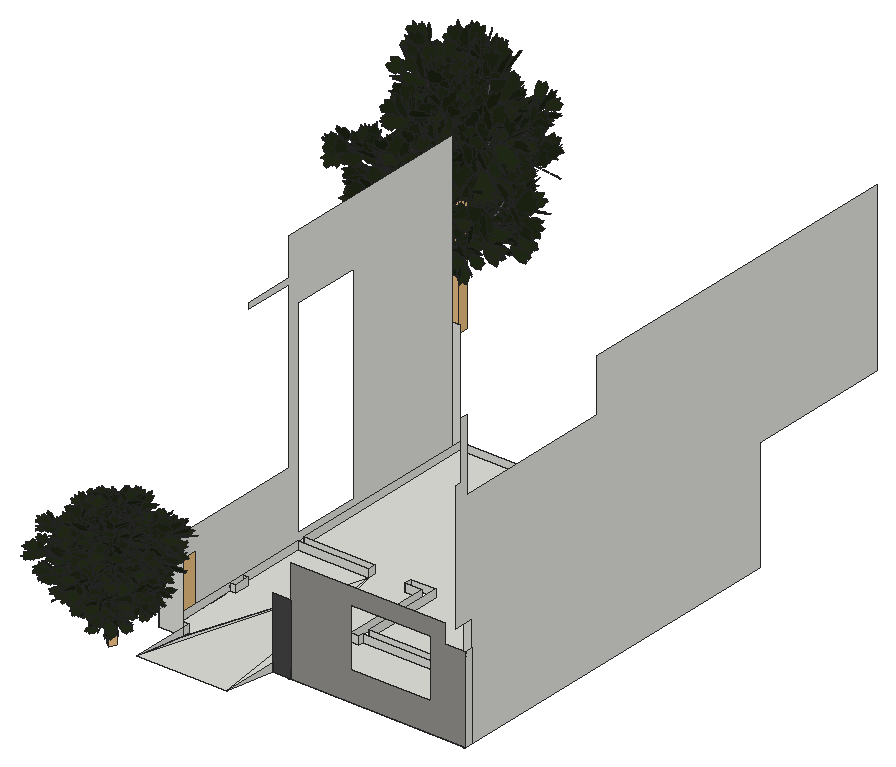
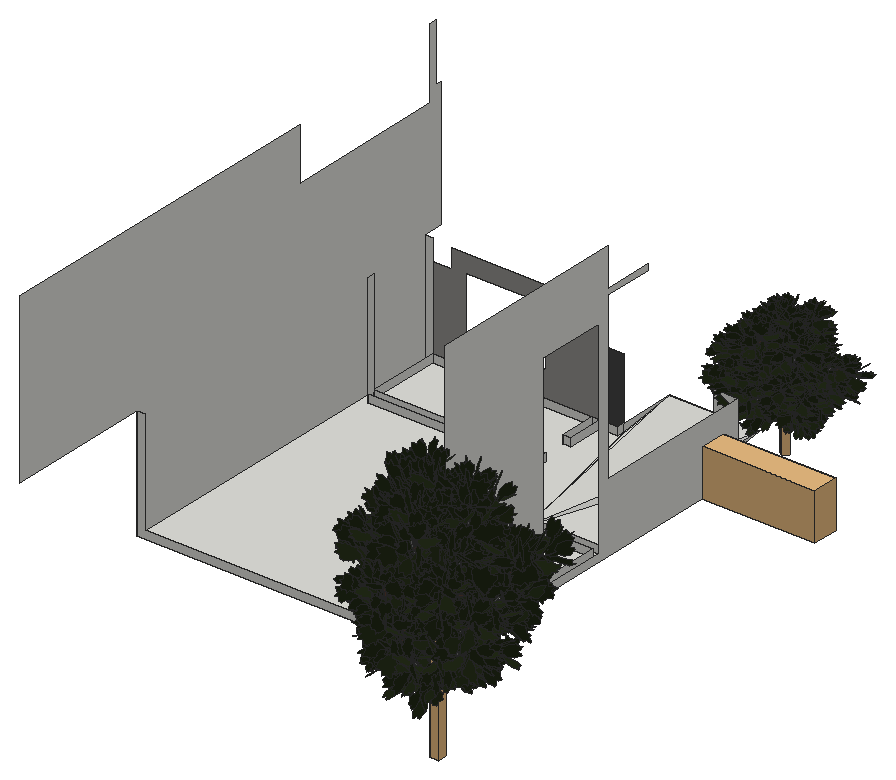
# SketchUp Ruby script. Lengths in inches.
U = 1.inch
M = Sketchup.active_model
def pt(a) = Geom::Point3d.new(a.map { |v| v * U })
def face(e, loops, mat)
  f = e.add_face(loops[0].map { |a| pt(a) })
  loops[1..].each { |l| e.add_face(l.map { |a| pt(a) }).erase! }
  f.material = f.back_material = mat if mat
  f
end
# faces: each face lists its corners as indices into pts; further lists are holes
def faces(e, pts, list, mat = nil) = list.each { |f| face(e, (f[0].is_a?(Array) ? f : [f]).map { |l| l.map { |i| pts[i] } }, mat) }
# xy, xz, yz: faces in a plane at the given z, y or x. An outline is a flat list of corners, or four numbers for a rectangle; further outlines are holes
def ring(l) = l.size == 4 ? [[l[0], l[1]], [l[2], l[1]], [l[2], l[3]], [l[0], l[3]]] : l.each_slice(2).to_a
def flat(e, list, mat, &to3) = list.each { |f| face(e, (f[0].is_a?(Array) ? f : [f]).map { |l| ring(l).map { |u, v| to3.(u, v) } }, mat) }
def xy(e, z, list, mat = nil) = flat(e, list, mat) { |x, y| [x, y, z] }
def xz(e, y, list, mat = nil) = flat(e, list, mat) { |x, z| [x, y, z] }
def yz(e, x, list, mat = nil) = flat(e, list, mat) { |y, z| [x, y, z] }
def lines(e, pts, list) = list.each { |a, b| e.add_line(pt(pts[a]), pt(pts[b])) }
# prism: a flat outline (further loops are holes) pulled along v
def prism(e, loops, v, mat = nil)
  f = face(e, loops, mat); d = Geom::Vector3d.new(v.map { |x| x * U })
  f.pushpull(f.normal.samedirection?(d) ? d.length : -d.length)
end
def box(e, o, s, mat = nil) = prism(e, [[o, [o[0] + s[0], o[1], o[2]], [o[0] + s[0], o[1] + s[1], o[2]], [o[0], o[1] + s[1], o[2]]]], [0, 0, s[2]], mat)
def at(x, y, z, deg = 0) = Geom::Transformation.translation(pt([x, y, z])) * Geom::Transformation.rotation(ORIGIN, Z_AXIS, deg.degrees)
def axes(o, x, y, z) = Geom::Transformation.new([*x, 0, *y, 0, *z, 0, *pt(o).to_a, 1])
def part(name) = M.definitions.add(name)
# library, detail: a bought-in or finely detailed component or shape, given as its bounding box
def library(name, o, s) = part(name).tap { |d| box(d.entities, o, s) }
def detail(e, o, s) = box(e.add_group.entities, o, s)
def put(e, d, t, mat = nil) = e.add_instance(d, t).tap { |i| i.material = mat if mat }
def group(e, t, mat = nil) = e.add_group.tap { |g| g.transformation = t; g.material = mat if mat }.entities
root = M.entities
M.materials.add("Green ash – green texture").color = [33, 41, 22]
M.materials.add("[Color_005]1").color = [114, 114, 114]
M.materials.add("[Color_D09]1").color = [86, 59, 49]
M.materials.add("[Granite Dark Gray]").color = [69, 68, 68]
M.materials.add("[Granite Light Gray]").color = [149, 148, 144]
c1 = library("Tree trunk",[-6.35,9.4375,-76.57],[12.56,13.68,315.77])
c2 = part("Component\#32")
xz(c2.entities,0,[[2.54,0,9.87,0.64,10.99,2.07,11.4,3.42,15.13,2.28,14.48,4.31,16.14,5.21,16.14,6.08,19.81,7.28,19.6,9.67,17.45,11.49,17.45,12.16,18.82,14.37,17.48,14.37,14.41,13.66,14.41,15.23,12.5625,17.49,9.84,15.21,8.9,13.85,7.74,13.625,7.35,12.68,6.87,13.02,6.35,12.27,5.92,10.47,4.2,7.42,2.84,6.89,0,2.38,0.07,1.59,2.8125,4.94,3.37,3.59,2.54,3.37,2.12,2.22]],"Green ash – green texture")
c3 = part("Component\#31")
xz(c3.entities,0,[[1.1,0,1.61,0,2.73,1.11,4.34,2.72,5.21,6.36,5.85,7.16,6.35,6.9375,6.85,8.05,8.03,8.05,8.625,9.25,10.11,11.7,9.56,13.83,9.56,15.84,7.83,15.84,6.03,14.37,5.31,16.54,4.4375,17.39,1.45,14.31,0,9.15,1.4,5.18,3.01,6.08,1.98,1.39]],"Green ash – green texture")
c4 = part("Component\#30")
put(c4.entities,c2,axes([0,7.77,0],[1,0,0],[0,0.89571,0.44464],[0,-0.44464,0.89571]))
put(c4.entities,c3,axes([2.15,6.37,5.26],[0.57629,-0.80824,0.12095],[0.79263,0.51673,-0.3236],[0.19905,0.28236,0.93843]))
c5 = part("Component\#33")
put(c5.entities,c4,axes([-4.97,-3.22,4.05],[0.69883,-0.69034,0.18725],[0.53248,0.3273,-0.7806],[0.47759,0.64522,0.59632]))
c6 = part("Component\#35")
put(c6.entities,c5,axes([0,5.2,2.2],[1,0,0],[0,0.90259,0.43051],[0,-0.43051,0.90259]))
c7 = part("leaf group 2")
put(c7.entities,c6,axes([-11.99,4.41,-4.35],[2.22014,-0.82385,1.14017],[1.36501,1.77637,-1.37441],[-0.33979,1.75315,1.92841]))
c8 = part("Component\#37")
put(c8.entities,c7,axes([-5.27,11.65,1.68],[-0.48323,0.10636,-0.43072],[-0.11515,-0.64511,-0.03012],[-0.42845,0.05342,0.49388]))
c9 = part("Component\#36")
xz(c9.entities,0,[[0.64,0,0,0.1875,4.21,2.81,8.59,4.11,12.8,4.11,19.57,2.81,12.8,3.73,8.59,3.73,4.21,2.3125]],"[Color_D09]1")
c10 = part("Leaf cluster")
put(c10.entities,c8,axes([23.53,12.57,24.85],[0.06536,-0.90475,-0.42089],[0.61791,-0.2945,0.72901],[-0.78353,-0.30772,0.53981]))
put(c10.entities,c8,axes([22.7,12.25,24.83],[-0.47146,-0.89493,0.11311],[0.80135,-0.48549,-0.35888],[0.36776,-0.0521,0.90651]))
put(c10.entities,c8,axes([24.25,0.65,20.83],[0.8253,-0.50372,0.24924],[0.23848,0.71461,0.65749],[-0.51157,-0.48438,0.71194]))
put(c10.entities,c8,axes([23.54,-2.45,18.63],[0.04689,-0.92492,0.3511],[0.72122,-0.28285,-0.64421],[0.71641,0.2674,0.65188]))
put(c10.entities,c8,axes([22.39,16.15,27.04],[-0.5311,-0.82173,0.2419],[0.41574,0.01583,0.89559],[-0.77461,0.50499,0.40813]))
put(c10.entities,c9,axes([22.76,-5.09,13.48],[0,1.66539,0.44624],[-1.72414,0,0],[0,-0.44624,1.66539]))
c11 = part("Bare twig")
p = [[0,0,0.13],[0.41,0.77,0],[4.07,2.79,10.125],[3.73,2.15,10.23],[7.66,4.77,23.875],[7.4,4.27,23.96],
  [8.6875,5.26,35.99],[8.5,4.91,36.05],[8.32,4.9375,46.95],[8.21,4.74,46.98]]
faces(c11.entities,p,[[0,1,2,3],[3,2,4,5],[4,6,7,5],[6,8,9,7]],"[Color_005]1")
c12 = part("Leafy twig")
put(c12.entities,c11,axes([3.13,0.17,-0.45],[3.38032,6.88592,0.52481],[-5.85488,3.97559,0.303],[0,-1.35912,3.54524]))
put(c12.entities,c8,axes([0.37,31.375,148.94],[0.47772,0.64064,-1.51139],[2.85768,-0.62659,0.20284],[-0.43926,-3.3797,-0.3241]))
c13 = part("Leafy branch \#2")
put(c13.entities,c10,axes([-3.64,36.17,23.18],[0.95801,0.10249,0.26779],[-0.28581,0.41631,0.86313],[-0.02302,-0.90343,0.42812]))
put(c13.entities,c10,axes([13.16,55.79,39.92],[0.70711,-0.61725,0.34497],[0,0.48786,0.87292],[-0.70711,-0.61725,0.34497]))
put(c13.entities,c12,axes([18.8125,5.17,0.46],[0.25503,0,0],[0,0.20007,-0.0752],[0,0.16866,0.44872]))
put(c13.entities,c10,axes([23.62,-10.17,21.5],[-0.56253,0.81775,0.12181],[0.38738,0.13053,0.91263],[0.73041,0.56057,-0.39021]))
put(c13.entities,c10,axes([45.18,27.18,68.96],[-0.96593,-0.22593,0.12627],[0.12295,0.02876,0.992],[-0.22775,0.97372,0]))
c14 = part("Leafy branch")
put(c14.entities,c10,axes([28.11,72.66,46.26],[0.77413,-0.41274,-0.47998],[0.6311,0.56229,0.53435],[0.04934,-0.71657,0.69577]))
put(c14.entities,c10,axes([31.25,3.94,9.17],[0.73236,0.67893,0.05208],[-0.46223,0.55185,-0.69413],[-0.5,0.48428,0.71797]))
put(c14.entities,c10,axes([20.16,84.84,57.95],[0.96628,0.19619,0.16678],[-0.2575,0.73909,0.62245],[-0.00115,-0.6444,0.76469]))
put(c14.entities,c10,axes([30.13,29.18,11.93],[0.86603,0.2796,0.41452],[0,0.82904,-0.55919],[-0.5,0.48428,0.71797]))
put(c14.entities,c10,axes([47.67,28.63,-3.7],[0.1205,-0.71255,0.69119],[0.96646,0.24327,0.08231],[-0.2268,0.65809,0.71797]))
put(c14.entities,c10,axes([48.76,50.64,76.31],[-0.6716,0.46861,-0.57389],[0.01402,0.78248,0.62252],[0.74078,0.41004,-0.53209]))
put(c14.entities,c12,axes([42.34,0,10.34],[0.39368,0,0],[0,0.22544,-0.24092],[0,0.54032,0.50562]))
put(c14.entities,c10,axes([64.51,80.82,101.08],[-0.99604,0.06562,-0.06004],[-0.0106,0.58266,0.81265],[0.08831,0.81006,-0.57966]))
c15 = part("Leafy branch \#1")
put(c15.entities,c10,axes([26.17,74.02,40.56],[0.25882,-0.64004,0.72344],[0,0.74896,0.66262],[-0.96593,-0.1715,0.19384]))
put(c15.entities,c10,axes([6.38,24.03,55.81],[-0.04786,0.8645,-0.50035],[0.15558,0.50126,0.85119],[0.98666,-0.03711,-0.15849]))
put(c15.entities,c12,axes([17.68,0,1.01],[0.32282,0,0],[0,0.21407,-0.16545],[0,0.37107,0.48011]))
put(c15.entities,c10,axes([-9.1875,31.15,28.07],[0.82314,0.37626,-0.42529],[0,0.74896,0.66262],[0.56784,-0.54543,0.61649]))
put(c15.entities,c10,axes([0.54,-12.07,9.94],[0.19622,0.90478,-0.37799],[-0.67396,0.40444,0.61823],[0.71224,0.13344,0.68914]))
put(c15.entities,c10,axes([7.34,9.15,39.57],[0.05153,0.73872,-0.67204],[0.38679,0.60565,0.6954],[0.92072,-0.29578,-0.25452]))
put(c15.entities,c10,axes([36.2,51.23,15.73],[-0.18626,-0.35374,0.91661],[-0.31641,0.90483,0.2849],[-0.93016,-0.23696,-0.28046]))
c16 = part("Leafy branch \#3")
put(c16.entities,c12,axes([21.47,3.93,0.22],[0.25503,0,0],[0,0.21068,-0.03601],[0,0.08077,0.47252]))
put(c16.entities,c10,axes([-4.05,13.6875,55.34],[0.70711,0.70373,-0.069],[0,0.09758,0.99523],[0.70711,-0.70373,0.069]))
put(c16.entities,c10,axes([6.52,33.54,18.07],[0.92587,-0.37604,0.03687],[0,0.09758,0.99523],[-0.37784,-0.92145,0.09035]))
c17 = part("Green Ash")
put(c17.entities,c1,axes([99.99,94.03,63.71],[0.79573,0,0],[0,0.79573,0],[0,0,0.83213]))
put(c17.entities,c13,axes([101.67,85.93,193.17],[0.07998,0.81569,0],[-0.81569,0.07998,0],[0,0,0.89336]))
put(c17.entities,c13,axes([89.02,118.86,194.23],[0,-0.81737,0],[0.81737,0,0],[0,0,0.89093]))
put(c17.entities,c14,axes([137.88,109.2,140.96],[-0.78759,-0.14066,-0.22296],[0.03147,-0.75159,0.31311],[-0.21191,0.33708,0.76893]))
put(c17.entities,c14,axes([67.1875,107.625,70.5],[0.79573,0,0],[0,0.79193,0.11835],[0,-0.16418,0.84696]))
put(c17.entities,c14,axes([104.58,73.13,95.39],[-0.14386,0.73191,-0.43628],[-0.81295,0,0.24048],[0.24918,0.42257,0.75566]))
put(c17.entities,c14,axes([128.33,85.59,105.66],[-0.68407,0.52018,0],[-0.52018,-0.68407,0],[0,0,0.93673]))
put(c17.entities,c14,axes([128.77,118.32,82.77],[-0.64576,-0.27079,0],[0.27079,-0.64576,0],[0,0,0.76326]))
put(c17.entities,c13,axes([114.32,106.07,192.67],[-0.76861,0.19684,-0.06056],[-0.19893,-0.77561,0.00374],[-0.0533,0.05621,0.85925]))
put(c17.entities,c14,axes([83.56,80.16,142.32],[0.31858,0.60462,-0.23671],[-0.62954,0.35865,0.06881],[0.21751,0.1725,0.73337]))
put(c17.entities,c13,axes([81.16,104.7,186.36],[0.7834,-0.13954,0],[0.13954,0.7834,0],[0,0,0.86734]))
put(c17.entities,c15,axes([97.7,92.8125,165.31],[0,0.90235,0],[-0.8655,0,0.25525],[0.27822,0,0.94339]))
put(c17.entities,c14,axes([87.68,137.07,132.52],[0.23821,-0.65607,-0.06135],[0.65299,0.22764,0.12002],[-0.08486,-0.08995,0.75126]))
put(c17.entities,c16,axes([89.6875,123.91,227.86],[0.39786,-0.68912,0],[0.68912,0.39786,0],[0,0,0.86734]))
put(c17.entities,c14,axes([95.07,144,73.32],[0.17556,-0.89482,0],[0.86433,0.16957,0.23601],[-0.25244,-0.04953,0.96008]))
put(c17.entities,c16,axes([110.1,95.2,218.26],[-0.45054,0.64862,0.09741],[-0.63397,-0.46095,0.13707],[0.18329,0,0.84775]))
put(c17.entities,c15,axes([90.03,118.62,161.33],[0.51503,-0.86951,-0.19982],[0.85825,0.4318,0.39581],[-0.23035,-0.33528,1.02798]))
put(c17.entities,c15,axes([83.38,108.05,173.27],[0.82756,0,0],[0,0.81825,0.12375],[0,-0.13489,0.89189]))
put(c17.entities,c15,axes([111.27,114.42,147],[-0.60244,-0.5209,0.41631],[0.61593,-0.62057,0.13644],[0.19452,0.35171,0.8573]))
put(c17.entities,c14,axes([126.43,83.55,60.6],[-0.64533,0.52071,0.15494],[-0.51656,-0.64172,0.07919],[0.23936,-0.05752,0.84432]))
put(c17.entities,c15,axes([111.89,112.18,157.4375],[-0.70287,-0.34493,-0.15481],[0.28133,-0.68912,0.30665],[-0.24495,0.19829,0.79642]))
put(c17.entities,c14,axes([72.73,119.08,126.01],[0.66249,-0.22682,0],[0.22682,0.66249,0],[0,0,0.76326]))
c18 = part("Tree")
put(c18.entities,c14,axes([209.16,146.26,190.79],[-0.28773,1.46382,-0.87256],[-1.6259,0,0.48096],[0.49836,0.84514,1.51132]))
put(c18.entities,c14,axes([134.38,215.25,141.01],[1.59145,0,0],[0,1.58386,0.23671],[0,-0.32836,1.69393]))
put(c18.entities,c13,axes([178.04,237.71,388.46],[0,-1.63474,0],[1.63474,0,0],[0,0,1.78187]))
put(c18.entities,c14,axes([256.65,171.18,211.31],[-1.36815,1.04036,0],[-1.04036,-1.36815,0],[0,0,1.87346]))
put(c18.entities,c14,axes([167.11,160.33,284.63],[0.63716,1.20925,-0.47341],[-1.25908,0.71729,0.13762],[0.43501,0.34501,1.46674]))
put(c18.entities,c1,axes([199.97,188.06,127.43],[1.59145,0,0],[0,1.59145,0],[0,0,1.66425]))
put(c18.entities,c14,axes([275.77,218.4,281.93],[-1.57517,-0.28132,-0.44593],[0.06295,-1.50318,0.62621],[-0.42383,0.67416,1.53786]))
put(c18.entities,c14,axes([190.14,288,146.64],[0.35111,-1.78964,0],[1.72866,0.33915,0.47202],[-0.50488,-0.09905,1.92016]))
put(c18.entities,c14,axes([257.54,236.65,165.53],[-1.29152,-0.54158,0],[0.54158,-1.29152,0],[0,0,1.52652]))
put(c18.entities,c14,axes([175.36,274.13,265.04],[0.47642,-1.31213,-0.12271],[1.30597,0.45529,0.24003],[-0.16973,-0.17989,1.50253]))
put(c18.entities,c13,axes([228.65,212.14,385.35],[-1.53723,0.39369,-0.12111],[-0.39786,-1.55122,0.00748],[-0.10661,0.11241,1.71849]))
put(c18.entities,c16,axes([179.375,247.82,455.73],[0.79573,-1.37824,0],[1.37824,0.79573,0],[0,0,1.73468]))
put(c18.entities,c16,axes([220.2,190.4,436.52],[-0.90108,1.29724,0.19482],[-1.26794,-0.9219,0.27414],[0.36658,0,1.69551]))
put(c18.entities,c15,axes([195.4,185.625,330.61],[0,1.80471,0],[-1.731,0,0.5105],[0.55644,0,1.88679]))
put(c18.entities,c15,axes([180.07,237.23,322.66],[1.03006,-1.73903,-0.39964],[1.71651,0.8636,0.79163],[-0.4607,-0.67055,2.05597]))
put(c18.entities,c14,axes([252.86,167.09,121.2],[-1.29065,1.04142,0.30989],[-1.03312,-1.28343,0.15838],[0.47872,-0.11505,1.68865]))
put(c18.entities,c14,axes([145.45,238.15,252.03],[1.32497,-0.45364,0],[0.45364,1.32497,0],[0,0,1.52652]))
put(c18.entities,c15,axes([222.54,228.83,294],[-1.20488,-1.04179,0.83261],[1.23186,-1.24114,0.27288],[0.38905,0.70343,1.7146]))
put(c18.entities,c15,axes([223.77,224.36,314.875],[-1.40575,-0.68986,-0.30962],[0.56266,-1.37824,0.6133],[-0.4899,0.39658,1.59284]))
put(c18.entities,c15,axes([166.75,216.1,346.53],[1.65511,0,0],[0,1.6365,0.2475],[0,-0.26977,1.78379]))
put(c18.entities,c13,axes([162.33,209.39,372.71],[1.56679,-0.27909,0],[0.27909,1.56679,0],[0,0,1.73468]))
put(c18.entities,c13,axes([203.35,171.86,386.35],[0.15996,1.63137,0],[-1.63137,0.15996,0],[0,0,1.78672]))
c19 = library("Su Tree",[-11.31,-37.43,0],[22.62,74.86,25.7])
xy(root,-9,[[219.74,317.12,219.74,739.58,229.21,739.58,229.21,514.52,310.83,514.52,310.83,505.52,229.21,505.52,229.21,325.52,247.49,325.52,247.49,317.12],[247.49,317.12,247.49,325.52,229.21,325.52,229.21,408.6,235.21,408.6,235.21,426.23,229.21,426.23,229.21,505.52,310.83,505.52],[351.06,317.12,310.83,505.52,310.83,514.52,229.21,514.52,229.21,739.58,574.21,739.58,574.21,325.52,565.21,325.52,565.21,418.52,381.21,418.52,381.21,514.52,352.83,514.52,352.83,505.52,372.21,505.52,372.21,403.52,381.21,403.52,381.21,409.52,565.21,409.52,565.21,325.52,381.21,325.52,381.21,367.52,372.21,367.52,372.21,325.52,351.48,325.52,351.48,317.12],[247.49,317.12,310.83,505.52,351.06,317.12],[351.48,317.12,372.21,317.13],
  [351.48,317.13,574.21,325.52],[372.21,325.52,381.21,367.52]])
xy(root,-9,[[372.21,317.12,574.21,317.13]],"[Granite Light Gray]")
xz(root,317.12,[[219.74,-9,247.49,72],[351.06,-9,351.48,0]])
xz(root,317.12,[[351.48,-9,372.21,72]],"[Granite Dark Gray]")
xz(root,317.13,[[[372.21,-9,574.21,-9,574.21,89.8125,549.96,89.8125,549.96,111.01,372.21,111.01],[441.07,24.15,532.88,91.74]]],"[Granite Light Gray]")
xz(root,325.52,[[229.21,-9,247.49,0],[351.48,-9,372.21,0],[372.21,-9,381.21,0],[381.21,-9,565.21,0],[565.21,-9,574.21,120]])
xz(root,367.52,[[372.21,-9,381.21,0]])
xz(root,403.52,[[372.21,-9,381.21,0]])
xz(root,408.6,[[229.21,-9,235.21,0]])
xz(root,409.52,[[381.21,-9,565.21,0]])
xz(root,418.52,[[381.21,-9,565.21,0]])
xz(root,426.23,[[229.21,-9,235.21,0]])
xz(root,505.52,[[229.21,-9,310.83,0],[352.83,-9,372.21,0]])
xz(root,514.52,[[229.21,-9,310.83,0],[352.83,-9,381.21,0]])
xz(root,739.58,[[219.74,-9,229.21,120],[229.21,-9,229.21,0,565.21,0,565.21,120,574.21,120,574.21,-9]])
yz(root,219.74,[[[317.12,-9,317.12,72,505.52,72,505.52,261.3125,447.9375,261.3125,447.9375,268,505.52,268,505.52,312,739.58,312,739.58,-9],[518.03,0,597.83,237.3]]])
yz(root,229.21,[[325.52,-9,408.6,0],[408.6,-9,426.23,0],[426.23,-9,505.52,0],[514.52,-9,739.58,0]])
yz(root,235.21,[[408.6,-9,426.23,0]])
yz(root,247.49,[[317.12,-9,251,0,317.12,0],[317.12,-9,325.52,0]])
yz(root,310.83,[[505.52,-9,514.52,0]])
yz(root,351.06,[[317.12,-9,317.12,0,251,0]])
yz(root,351.48,[[317.12,-9,325.52,0]])
yz(root,352.83,[[505.52,-9,514.52,0]])
yz(root,372.21,[[325.52,-9,367.52,0],[403.52,-9,505.52,0]])
yz(root,372.21,[[317.12,-9,317.13,0]],"[Granite Light Gray]")
yz(root,381.21,[[325.52,-9,367.52,0],[403.52,-9,409.52,0],[418.52,-9,514.52,0]])
yz(root,565.21,[[325.52,-9,409.52,0],[409.52,-9,418.52,120]])
yz(root,574.21,[[325.52,-9,739.58,-9,739.58,120,907.52,120,907.52,312,505.52,312,505.52,252,317.26,252,317.26,334.1875,309.07,334.1875,309.07,268,302.12,268,302.12,120,325.52,120],[317.13,-9,325.52,89.8125]])
yz(root,574.21,[[317.12,-9,317.13,89.8125]],"[Granite Light Gray]")
p = [[247.49,251,0],[247.49,317.12,-9],[310.83,505.52,-9],[351.06,251,0],[351.06,317.12,-9]]
faces(root,p,[[0,1,2],[3,0,2],[1,4,3,0],[4,3,2]])
put(root,c17,at(0,791.82,0))
put(root,c18,axes([235.32,153.33,-5.27],[0.21238,0.31486,0],[-0.31486,0.21238,0],[0,0,0.24633]))
put(root,c19,axes([154.67,354.31,-9],[0,-1.3,0],[1.7387,0,0],[0,0,2.12]))
